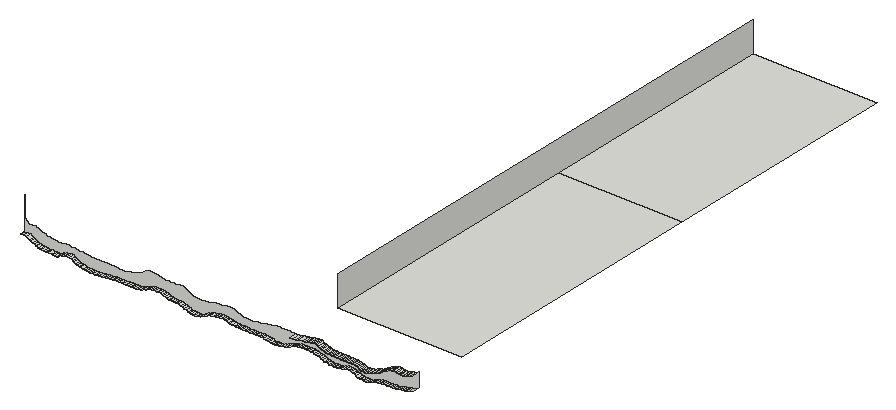
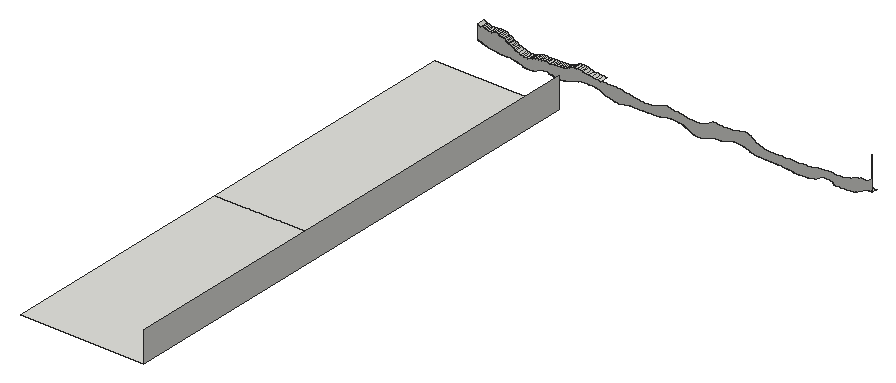
# SketchUp Ruby script. Lengths in inches.
U = 1.inch
M = Sketchup.active_model
def pt(a) = Geom::Point3d.new(a.map { |v| v * U })
def face(e, loops, mat)
  f = e.add_face(loops[0].map { |a| pt(a) })
  loops[1..].each { |l| e.add_face(l.map { |a| pt(a) }).erase! }
  f.material = f.back_material = mat if mat
  f
end
# faces: each face lists its corners as indices into pts; further lists are holes
def faces(e, pts, list, mat = nil) = list.each { |f| face(e, (f[0].is_a?(Array) ? f : [f]).map { |l| l.map { |i| pts[i] } }, mat) }
# xy, xz, yz: faces in a plane at the given z, y or x. An outline is a flat list of corners, or four numbers for a rectangle; further outlines are holes
def ring(l) = l.size == 4 ? [[l[0], l[1]], [l[2], l[1]], [l[2], l[3]], [l[0], l[3]]] : l.each_slice(2).to_a
def flat(e, list, mat, &to3) = list.each { |f| face(e, (f[0].is_a?(Array) ? f : [f]).map { |l| ring(l).map { |u, v| to3.(u, v) } }, mat) }
def xy(e, z, list, mat = nil) = flat(e, list, mat) { |x, y| [x, y, z] }
def xz(e, y, list, mat = nil) = flat(e, list, mat) { |x, z| [x, y, z] }
def yz(e, x, list, mat = nil) = flat(e, list, mat) { |y, z| [x, y, z] }
def lines(e, pts, list) = list.each { |a, b| e.add_line(pt(pts[a]), pt(pts[b])) }
# prism: a flat outline (further loops are holes) pulled along v
def prism(e, loops, v, mat = nil)
  f = face(e, loops, mat); d = Geom::Vector3d.new(v.map { |x| x * U })
  f.pushpull(f.normal.samedirection?(d) ? d.length : -d.length)
end
def box(e, o, s, mat = nil) = prism(e, [[o, [o[0] + s[0], o[1], o[2]], [o[0] + s[0], o[1] + s[1], o[2]], [o[0], o[1] + s[1], o[2]]]], [0, 0, s[2]], mat)
def at(x, y, z, deg = 0) = Geom::Transformation.translation(pt([x, y, z])) * Geom::Transformation.rotation(ORIGIN, Z_AXIS, deg.degrees)
def axes(o, x, y, z) = Geom::Transformation.new([*x, 0, *y, 0, *z, 0, *pt(o).to_a, 1])
def part(name) = M.definitions.add(name)
# library, detail: a bought-in or finely detailed component or shape, given as its bounding box
def library(name, o, s) = part(name).tap { |d| box(d.entities, o, s) }
def detail(e, o, s) = box(e.add_group.entities, o, s)
def put(e, d, t, mat = nil) = e.add_instance(d, t).tap { |i| i.material = mat if mat }
def group(e, t, mat = nil) = e.add_group.tap { |g| g.transformation = t; g.material = mat if mat }.entities
root = M.entities
xy(root,237.65,[[2039.58,566.68,2040.27,568.68],[2040.27,566.68,2040.89,568.68]])
xy(root,238.18,[[2133.53,566.68,2134.21,568.68]])
xy(root,238.33,[[2048.68,566.68,2049.23,568.68],[2049.23,566.68,2049.91,568.68]])
xy(root,238.34,[[2050.59,566.68,2051.52,568.68],[2051.52,566.68,2052.01,568.68],[2052.01,566.68,2052.77,568.68],[2052.77,566.68,2053.4,568.68],[2053.4,566.68,2054.15,568.68],
  [2054.15,566.68,2054.77,568.68],[2054.77,566.68,2055.54,568.68],[2055.54,566.68,2056.16,568.68]])
xy(root,238.62,[[2100.06,566.68,2100.83,568.68],[2100.83,566.68,2101.46,568.68],[2101.46,566.68,2102.22,568.68],[2102.22,566.68,2102.84,568.68],[2102.84,566.68,2103.69,568.68],
  [2103.69,566.68,2104.33,568.68],[2104.33,566.68,2104.95,568.68]])
xy(root,238.625,[[2098.64,566.68,2099.5,568.68]])
xy(root,238.89,[[2154.45,566.68,2155.13,568.68]])
xy(root,238.9,[[2155.89,566.68,2156.51,568.68],[2156.51,566.68,2157.28,568.68]])
xy(root,240.43,[[2122.73,566.68,2123.3,568.68]])
xy(root,241.52,[[2010.28,566.68,2010.34,568.68]])
xy(root,242.28,[[2140.55,565.74,2141.0625,568.68]])
xy(root,242.3,[[2138.79,565.74,2139.46,568.68]])
xy(root,242.33,[[2136.38,565.74,2136.96,568.68]])
xy(root,242.625,[[2115.89,589.83,2164.35,697.21],[2115.89,697.21,2164.35,792.52]])
xz(root,568.68,[[2079.2,236.98,2078.59,237.01,2077.9,237.04,2077.14,237.11,2076.45,237.2,2075.92,237.33,2075.25,237.68,2074.3125,237.96,2073.75,238.28,2072.97,238.43,2072.19,238.78,2071.52,238.79,2070.98,238.8,2070.22,238.83,2069.47,238.875,2068.9,238.94,2068.32,239.04,2067.66,239.29,2067.08,239.53,2066.55,239.7,2065.86,239.92,2065.23,240.11,2064.45,240.27,2063.83,240.25,2063.125,240.23,2062.36,240.19,2061.6875,240.12,2061.03,240.03,2060.39,239.85,2059.84,239.52,2059.28,239.35,2058.69,239.18,2058.18,238.86,2057.49,238.72,2056.67,238.59,2056.16,238.34,2050.59,238.34,2049.91,238.33,2048.68,238.33,2047.96,238.32,2047.11,238.3,2046.48,238.28,2045.73,238.26,2045.1,238.15,2044.34,238.13,2043.79,238.1,2042.9375,237.98,2042.32,237.94,2041.56,237.89,2040.89,237.65,2039.58,237.65,2038.89,237.66,2038.14,237.67,2037.54,237.68,2036.93,237.71,2036.22,237.76,2035.53,237.82,2034.87,237.9,2033.93,238.21,2033.46,238.31,2032.55,238.43,2031.9,238.74,2031.32,239.11,2030.74,239.38,2030.28,239.71,2029.58,240.11,2028.89,240.09,2028.23,240.05,2027.64,239.99,2026.91,239.88,2026.36,239.69,2025.78,239.55,2025.22,238.9375,2024.69,238.77,2023.95,238.79,2023.08,238.8,2022.57,238.82,2021.53,238.92,2020.84,238.93,2020.14,238.94,2019.44,238.97,2018.76,239.03,2018.07,239.09,2017.29,239.19,2016.78,239.52,2016.22,239.64,2015.77,239.86,2014.98,240.2,2014.38,240.59,2013.84,240.85,2012.82,241.55,2011.55,241.69,2010.34,241.52,2010.34,246.2,2011.91,244.96,2013.3,244.9375,2014.55,244.92,2014.77,244.61,2015.33,244.54,2016.09,244.41,2016.76,244.11,2017.28,243.95,2017.94,243.79,2018.46,243.48,2019.1,243.3,2019.6875,243.14,2020.17,243.06,2020.89,242.85,2021.47,242.78,2022.28,242.73,2022.82,242.68,2023.49,242.51,2024.01,242.46,2024.55,242.58,2025.18,242.57,2025.81,242.81,2026.38,242.86,2026.94,242.89,2027.58,242.92,2028.01,242.625,2028.62,242.65,2029.17,242.62,2029.8,242.58,2030.36,242.57,2031,242.48,2031.66,242.38,2032.32,242.34,2032.99,242.24,2034.16,241.96,2034.93,241.89,2035.75,241.83,2036.35,241.78,2037.12,241.75,2037.57,241.74,2038.12,241.72,2039.38,241.7,2040.11,241.69,2040.78,241.68,2041.37,241.68,2041.86,241.67,2042.5625,241.74,2043.13,241.75,2045.13,241.75,2045.62,241.67,2046.15,241.66,2046.76,241.57,2047.3,241.53,2047.92,241.51,2048.47,241.49,2049.17,241.48,2049.83,241.47,2050.4,241.46,2051.11,241.6,2051.84,241.85,2052.51,241.91,2053.41,242.1,2054.18,242.46,2054.88,242.78,2055.65,242.97,2056.18,243.23,2056.58,243.48,2057.1,243.72,2057.4375,244.12,2057.91,244.39,2058.39,244.73,2058.875,244.87,2059.46,244.95,2060.14,245.01,2060.79,244.81,2061.36,244.7,2061.84,244.67,2062.45,244.55,2062.99,244.51,2063.45,244.25,2064.2,244.11,2064.76,244.04,2065.38,243.99,2066.1,243.95,2066.6,243.93,2067.29,243.91,2067.86,243.89,2068.56,243.88,2069.21,243.94,2069.85,243.95,2070.41,244.1,2071.04,244.13,2071.52,244.15,2072.04,244.17,2072.56,244.18,2073.16,243.8,2073.7,243.43,2074.31,243.09,2074.7,242.875,2075.2,242.68,2075.79,242.51,2076.3,242.21,2076.9,242.11,2077.58,241.96,2078.14,241.89,2078.6,241.85,2079.12,241.8125,2079.63,241.79,2080.21,241.78,2080.88,241.91,2081.35,241.93,2082.02,242.09,2082.79,242.2,2083.29,242.24,2083.9,242.42,2084.45,242.47,2085.2,242.71,2085.84,242.78,2086.32,242.82,2087.01,242.85,2087.71,242.87,2088.26,243.02,2088.88,243.05,2089.43,243.29,2090.11,243.35,2090.66,243.39,2091.26,243.42,2092.03,243.14,2092.6,242.9375,2093.15,242.65,2093.77,242.39,2094.53,242.14,2095.17,241.89,2095.66,241.78,2096.71,241.63,2097.48,241.56,2098.08,241.51,2098.53,241.48,2099.05,241.46,2099.92,241.51,2100.64,241.59,2101.58,241.82,2102.36,241.87,2103.125,241.98,2103.74,242.02,2104.39,242.19,2105.09,242.38,2105.58,242.4375,2106.1,242.48,2106.76,242.58,2107.29,242.61,2107.875,242.77,2108.33,242.95,2108.89,243.01,2109.4,243.05,2109.97,243.08,2110.625,243.09,2112.78,243.09,2113.35,243.08,2113.9375,243.07,2114.52,243.07,2115.18,243.0625,2115.79,243.05,2116.47,243.05,2117.74,243.1,2118.91,243.17,2120.05,243.4,2121.3125,243.52,2122.44,243.71,2123.34,243.99,2124.04,244.08,2124.74,244.21,2125.32,244.27,2125.86,244.3,2126.53,244.39,2127.125,244.19,2127.5,243.88,2127.98,243.59,2128.53,243.33,2129.08,243.22,2129.57,242.92,2130.05,242.75,2130.61,242.6,2131.17,242.52,2131.73,242.47,2132.3125,242.43,2132.89,242.4,2133.47,242.39,2134.05,242.37,2134.63,242.36,2135.22,242.35,2136.38,242.33,2136.96,242.33,2137.68,242.32,2138.15,242.3125,2138.79,242.3,2139.46,242.3,2139.91,242.29,2140.55,242.28,2141.0625,242.28,2141.69,242.2,2142.27,241.97,2142.84,241.84,2143.35,241.57,2143.77,241.33,2144.24,241.24,2144.77,241.17,2145.24,241.12,2145.84,241.09,2146.41,241.14,2147.05,241.35,2147.64,241.46,2148.58,241.85,2149.58,242.23,2150.14,242.42,2150.86,242.61,2151.375,242.91,2151.75,243.14,2152.29,243.52,2152.77,243.71,2153.1,244.02,2153.54,244.21,2154.13,244.57,2154.6,244.76,2155.22,245.125,2155.72,245.32,2156.2,245.41,2156.75,245.48,2157.24,245.59,2157.77,245.55,2158.38,245.35,2158.87,245.31,2159.42,245.27,2159.98,245.24,2160.54,245.22,2161.1,245.34,2161.73,245.42,2162.3125,245.52,2162.69,245.76,2163.16,245.9,2164.35,246.43,2164.35,240.89,2162.52,240.1,2161.96,239.96,2161.4375,239.81,2160.75,239.53,2160.2,239.49,2159.48,239.42,2158.68,239.28,2157.91,239.15,2157.28,238.9,2155.89,238.9,2155.13,238.89,2154.45,238.89,2153.77,238.88,2153.23,238.875,2152.47,238.86,2151.73,238.83,2151.16,238.8,2150.58,238.74,2149.92,238.6,2149.35,238.51,2148.82,238.33,2148.13,238.08,2147.45,237.84,2146.76,237.5625,2146.16,237.47,2145.48,237.4,2144.75,237.42,2144.18,237.45,2143.59,237.51,2142.99,237.59,2142.45,237.71,2141.62,238,2140.91,238.33,2140.36,238.57,2139.86,238.86,2139.34,238.96,2138.65,239.02,2137.97,239.125,2137.23,239.04,2136.66,238.66,2136.07,238.61,2135.41,238.55,2134.89,238.27,2134.21,238.18,2133.53,238.18,2132.86,238.11,2132.33,238.15,2131.51,238.19,2130.9375,238.26,2130.37,238.48,2129.71,238.56,2129.14,238.67,2128.62,239.01,2127.9375,239.18,2127.3125,239.5,2126.55,239.65,2125.9375,239.8,2125.18,239.96,2124.53,240.23,2123.95,240.27,2123.3,240.43,2122.73,240.43,2122.15,240.42,2121.625,240.41,2120.93,240.4,2120.24,240.37,2119.55,240.33,2118.87,240.27,2118.19,240.17,2117.57,239.97,2116.92,239.75,2116.18,239.375,2115.39,239.08,2114.51,238.72,2113.76,238.46,2112.54,238.14,2111.42,237.88,2110.77,237.87,2109.9,237.74,2109.19,237.79,2108.42,237.86,2107.79,238.15,2107.02,238.19,2106.4,238.25,2105.64,238.45,2104.95,238.62,2100.06,238.62,2099.5,238.625,2098.64,238.625,2097.95,238.63,2097.33,238.64,2096.55,238.65,2095.88,238.66,2095.19,238.6875,2094.52,238.73,2094.04,238.78,2093.16,238.93,2092.39,239.07,2091.84,239.16,2090.99,239.44,2090.32,239.56,2089.71,239.72,2088.98,239.7,2088.42,239.69,2087.83,239.65,2087.21,239.6,2086.72,239.54,2085.91,239.31,2084.91,239.22,2084.33,239.12,2083.6875,238.76,2083.05,238.51,2082.49,238.375,2082.05,238.02,2081.35,237.74,2080.73,237.43,2079.88,237.22],[2010.28,241.52,2010.34,254.5]])
yz(root,2115.89,[[589.83,242.625,792.52,254.5]])
p = [[2077.14,568.68,237.11],[2077.9,568.68,237.04],[2077.9,566.68,237.04],[2077.14,566.68,237.11],[2078.59,568.68,237.01],[2078.59,566.68,237.01],
  [2079.2,568.68,236.98],[2079.2,566.68,236.98],[2079.88,568.68,237.22],[2079.88,566.68,237.22],[2076.45,568.68,237.2],[2076.45,566.68,237.2],
  [2075.92,568.68,237.33],[2075.92,566.68,237.33],[2080.73,568.68,237.43],[2080.73,566.68,237.43],[2075.25,568.68,237.68],[2075.25,566.68,237.68],
  [2081.35,568.68,237.74],[2081.35,566.68,237.74],[2144.18,568.68,237.45],[2144.75,568.68,237.42],[2144.75,566.68,237.42],[2144.18,566.68,237.45],
  [2145.48,568.68,237.4],[2145.48,566.68,237.4],[2146.16,568.68,237.47],[2146.16,566.68,237.47],[2142.99,568.68,237.59],[2143.59,568.68,237.51],
  [2143.59,566.68,237.51],[2142.99,566.68,237.59],[2146.76,568.68,237.5625],[2146.76,566.68,237.5625],[2040.89,568.68,237.65],[2041.56,568.68,237.89],
  [2041.56,566.68,237.89],[2040.89,566.68,237.65],[2142.45,568.68,237.71],[2142.45,566.68,237.71],[2147.45,568.68,237.84],[2147.45,566.68,237.84],
  [2036.22,568.68,237.76],[2036.93,568.68,237.71],[2036.93,566.68,237.71],[2036.22,566.68,237.76],[2037.54,568.68,237.68],[2037.54,566.68,237.68],
  [2038.14,568.68,237.67],[2038.14,566.68,237.67],[2038.89,568.68,237.66],[2038.89,566.68,237.66],[2039.58,568.68,237.65],[2039.58,566.68,237.65],
  [2074.3125,568.68,237.96],[2074.3125,566.68,237.96],[2082.05,568.68,238.02],[2082.05,566.68,238.02],[2109.19,568.68,237.79],[2109.9,568.68,237.74],
  [2109.9,566.68,237.74],[2109.19,566.68,237.79],[2110.77,568.68,237.87],[2110.77,566.68,237.87],[2141.62,568.68,238],[2141.62,566.68,238],
  [2034.87,568.68,237.9],[2035.53,568.68,237.82],[2035.53,566.68,237.82],[2034.87,566.68,237.9],[2108.42,568.68,237.86],[2108.42,566.68,237.86],
  [2148.13,568.68,238.08],[2148.13,566.68,238.08],[2033.93,568.68,238.21],[2033.93,566.68,238.21],[2042.32,568.68,237.94],[2042.32,566.68,237.94],
  [2042.9375,568.68,237.98],[2042.9375,566.68,237.98],[2107.79,568.68,238.15],[2107.79,566.68,238.15],[2111.42,568.68,237.88],[2111.42,566.68,237.88],
  [2112.54,568.68,238.14],[2112.54,566.68,238.14],[2043.79,568.68,238.1],[2043.79,566.68,238.1],[2073.75,568.68,238.28],[2073.75,566.68,238.28],
  [2082.49,568.68,238.375],[2082.49,566.68,238.375],[2140.91,568.68,238.33],[2140.91,566.68,238.33],[2044.34,568.68,238.13],[2044.34,566.68,238.13],
  [2045.1,568.68,238.15],[2045.1,566.68,238.15],[2107.02,568.68,238.19],[2107.02,566.68,238.19],[2113.76,568.68,238.46],[2113.76,566.68,238.46],
  [2131.51,568.68,238.19],[2132.33,568.68,238.15],[2132.33,566.68,238.15],[2131.51,566.68,238.19],[2132.86,568.68,238.11],[2132.86,566.68,238.11],
  [2133.53,568.68,238.18],[2133.53,566.68,238.18],[2148.82,568.68,238.33],[2148.82,566.68,238.33],[2033.46,568.68,238.31],[2033.46,566.68,238.31],
  [2045.73,568.68,238.26],[2045.73,566.68,238.26],[2106.4,568.68,238.25],[2106.4,566.68,238.25],[2130.9375,568.68,238.26],[2130.9375,566.68,238.26],
  [2134.21,568.68,238.18],[2134.89,568.68,238.27],[2134.89,566.68,238.27],[2134.21,566.68,238.18],[2032.55,568.68,238.43],[2032.55,566.68,238.43],
  [2046.48,568.68,238.28],[2046.48,566.68,238.28],[2047.11,568.68,238.3],[2047.11,566.68,238.3],[2047.96,568.68,238.32],[2047.96,566.68,238.32],
  [2048.68,568.68,238.33],[2048.68,566.68,238.33],[2049.91,568.68,238.33],[2050.59,568.68,238.34],[2050.59,566.68,238.34],[2049.91,566.68,238.33],
  [2056.16,568.68,238.34],[2056.67,568.68,238.59],[2056.67,566.68,238.59],[2056.16,566.68,238.34],[2072.97,568.68,238.43],[2072.97,566.68,238.43],
  [2105.64,568.68,238.45],[2105.64,566.68,238.45],[2130.37,568.68,238.48],[2130.37,566.68,238.48],[2135.41,568.68,238.55],[2135.41,566.68,238.55],
  [2140.36,568.68,238.57],[2140.36,566.68,238.57],[2149.35,568.68,238.51],[2149.35,566.68,238.51],[2031.9,568.68,238.74],[2031.9,566.68,238.74],
  [2072.19,568.68,238.78],[2072.19,566.68,238.78],[2083.05,568.68,238.51],[2083.05,566.68,238.51],[2083.6875,568.68,238.76],[2083.6875,566.68,238.76],
  [2104.95,568.68,238.62],[2104.95,566.68,238.62],[2114.51,568.68,238.72],[2114.51,566.68,238.72],[2129.71,568.68,238.56],[2129.71,566.68,238.56],
  [2136.07,568.68,238.61],[2136.07,566.68,238.61],[2149.92,568.68,238.6],[2149.92,566.68,238.6],[2057.49,568.68,238.72],[2057.49,566.68,238.72],
  [2095.88,568.68,238.66],[2096.55,568.68,238.65],[2096.55,566.68,238.65],[2095.88,566.68,238.66],[2097.33,568.68,238.64],[2097.33,566.68,238.64],
  [2097.95,568.68,238.63],[2097.95,566.68,238.63],[2098.64,568.68,238.625],[2098.64,566.68,238.625],[2099.5,568.68,238.625],[2100.06,568.68,238.62],
  [2100.06,566.68,238.62],[2099.5,566.68,238.625],[2129.14,568.68,238.67],[2129.14,566.68,238.67],[2136.66,568.68,238.66],[2136.66,566.68,238.66],
  [2139.86,568.68,238.86],[2139.86,566.68,238.86],[2150.58,568.68,238.74],[2150.58,566.68,238.74],[2031.32,568.68,239.11],[2031.32,566.68,239.11],
  [2058.18,568.68,238.86],[2058.18,566.68,238.86],[2094.04,568.68,238.78],[2094.52,568.68,238.73],[2094.52,566.68,238.73],[2094.04,566.68,238.78],
  [2095.19,568.68,238.6875],[2095.19,566.68,238.6875],[2115.39,568.68,239.08],[2115.39,566.68,239.08],[2128.62,568.68,239.01],[2128.62,566.68,239.01],
  [2137.23,568.68,239.04],[2137.23,566.68,239.04],[2151.16,568.68,238.8],[2151.16,566.68,238.8],[2021.53,568.68,238.92],[2022.57,568.68,238.82],
  [2022.57,566.68,238.82],[2021.53,566.68,238.92],[2023.08,568.68,238.8],[2023.08,566.68,238.8],[2023.95,568.68,238.79],[2023.95,566.68,238.79],
  [2024.69,568.68,238.77],[2024.69,566.68,238.77],[2025.22,568.68,238.9375],[2025.22,566.68,238.9375],[2069.47,568.68,238.875],[2070.22,568.68,238.83],
  [2070.22,566.68,238.83],[2069.47,566.68,238.875],[2070.98,568.68,238.8],[2070.98,566.68,238.8],[2071.52,568.68,238.79],[2071.52,566.68,238.79],
  [2084.33,568.68,239.12],[2084.33,566.68,239.12],[2093.16,568.68,238.93],[2093.16,566.68,238.93],[2151.73,568.68,238.83],[2151.73,566.68,238.83],
  [2152.47,568.68,238.86],[2152.47,566.68,238.86],[2019.44,568.68,238.97],[2020.14,568.68,238.94],[2020.14,566.68,238.94],[2019.44,566.68,238.97],
  [2020.84,568.68,238.93],[2020.84,566.68,238.93],[2025.78,568.68,239.55],[2025.78,566.68,239.55],[2058.69,568.68,239.18],[2058.69,566.68,239.18],
  [2068.32,568.68,239.04],[2068.9,568.68,238.94],[2068.9,566.68,238.94],[2068.32,566.68,239.04],[2092.39,568.68,239.07],[2092.39,566.68,239.07],
  [2139.34,568.68,238.96],[2139.34,566.68,238.96],[2153.23,568.68,238.875],[2153.23,566.68,238.875],[2153.77,568.68,238.88],[2153.77,566.68,238.88],
  [2154.45,568.68,238.89],[2154.45,566.68,238.89],[2155.13,568.68,238.89],[2155.89,568.68,238.9],[2155.89,566.68,238.9],[2155.13,566.68,238.89],
  [2157.28,568.68,238.9],[2157.91,568.68,239.15],[2157.91,566.68,239.15],[2157.28,566.68,238.9],[2018.07,568.68,239.09],[2018.76,568.68,239.03],
  [2018.76,566.68,239.03],[2018.07,566.68,239.09],[2067.66,568.68,239.29],[2067.66,566.68,239.29],[2127.9375,568.68,239.18],[2127.9375,566.68,239.18],
  [2137.97,568.68,239.125],[2137.97,566.68,239.125],[2138.65,568.68,239.02],[2138.65,566.68,239.02],[2017.29,568.68,239.19],[2017.29,566.68,239.19],
  [2030.74,568.68,239.38],[2030.74,566.68,239.38],[2084.91,568.68,239.22],[2084.91,566.68,239.22],[2091.84,568.68,239.16],[2091.84,566.68,239.16],
  [2116.18,568.68,239.375],[2116.18,566.68,239.375],[2016.78,568.68,239.52],[2016.78,566.68,239.52],[2059.28,568.68,239.35],[2059.28,566.68,239.35],
  [2085.91,568.68,239.31],[2085.91,566.68,239.31],[2090.99,568.68,239.44],[2090.99,566.68,239.44],[2127.3125,568.68,239.5],[2127.3125,566.68,239.5],
  [2158.68,568.68,239.28],[2158.68,566.68,239.28],[2067.08,568.68,239.53],[2067.08,566.68,239.53],[2086.72,568.68,239.54],[2086.72,566.68,239.54],
  [2159.48,568.68,239.42],[2159.48,566.68,239.42],[2030.28,568.68,239.71],[2030.28,566.68,239.71],[2059.84,568.68,239.52],[2059.84,566.68,239.52],
  [2090.32,568.68,239.56],[2090.32,566.68,239.56],[2116.92,568.68,239.75],[2116.92,566.68,239.75],[2160.2,568.68,239.49],[2160.2,566.68,239.49],
  [2016.22,568.68,239.64],[2016.22,566.68,239.64],[2060.39,568.68,239.85],[2060.39,566.68,239.85],[2066.55,568.68,239.7],[2066.55,566.68,239.7],
  [2087.21,568.68,239.6],[2087.21,566.68,239.6],[2126.55,568.68,239.65],[2126.55,566.68,239.65],[2160.75,568.68,239.53],[2160.75,566.68,239.53],
  [2161.4375,568.68,239.81],[2161.4375,566.68,239.81],[2015.77,568.68,239.86],[2015.77,566.68,239.86],[2026.36,568.68,239.69],[2026.36,566.68,239.69],
  [2087.83,568.68,239.65],[2087.83,566.68,239.65],[2088.42,568.68,239.69],[2088.42,566.68,239.69],[2089.71,568.68,239.72],[2089.71,566.68,239.72],
  [2026.91,568.68,239.88],[2026.91,566.68,239.88],[2029.58,568.68,240.11],[2029.58,566.68,240.11],[2065.86,568.68,239.92],[2065.86,566.68,239.92],
  [2088.98,568.68,239.7],[2088.98,566.68,239.7],[2117.57,568.68,239.97],[2117.57,566.68,239.97],[2125.9375,568.68,239.8],[2125.9375,566.68,239.8],
  [2061.03,568.68,240.03],[2061.03,566.68,240.03],[2125.18,568.68,239.96],[2125.18,566.68,239.96],[2161.96,568.68,239.96],[2161.96,566.68,239.96],
  [2014.98,568.68,240.2],[2014.98,566.68,240.2],[2027.64,568.68,239.99],[2027.64,566.68,239.99],[2065.23,568.68,240.11],[2065.23,566.68,240.11],
  [2028.23,568.68,240.05],[2028.23,566.68,240.05],[2028.89,568.68,240.09],[2028.89,566.68,240.09],[2061.6875,568.68,240.12],[2061.6875,566.68,240.12],
  [2118.19,568.68,240.17],[2118.19,566.68,240.17],[2124.53,568.68,240.23],[2124.53,566.68,240.23],[2162.52,568.68,240.1],[2162.52,566.68,240.1],
  [2062.36,568.68,240.19],[2062.36,566.68,240.19],[2064.45,568.68,240.27],[2064.45,566.68,240.27],[2164.35,568.68,240.89],[2164.35,566.68,240.89],
  [2014.38,568.68,240.59],[2014.38,566.68,240.59],[2063.125,568.68,240.23],[2063.125,566.68,240.23],[2063.83,568.68,240.25],[2063.83,566.68,240.25],
  [2118.87,568.68,240.27],[2118.87,566.68,240.27],[2123.95,568.68,240.27],[2123.95,566.68,240.27],[2119.55,568.68,240.33],[2119.55,566.68,240.33],
  [2120.24,568.68,240.37],[2120.24,566.68,240.37],[2123.3,568.68,240.43],[2123.3,566.68,240.43],[2120.93,568.68,240.4],[2120.93,566.68,240.4],
  [2121.625,568.68,240.41],[2121.625,566.68,240.41],[2122.15,568.68,240.42],[2122.15,566.68,240.42],[2122.73,568.68,240.43],[2122.73,566.68,240.43],
  [2013.84,568.68,240.85],[2013.84,566.68,240.85],[2012.82,568.68,241.55],[2012.82,566.68,241.55],[2144.77,568.68,241.17],[2145.24,568.68,241.12],
  [2145.24,565.74,241.12],[2144.77,565.74,241.17],[2145.84,568.68,241.09],[2145.84,565.74,241.09],[2146.41,568.68,241.14],[2146.41,565.74,241.14],
  [2147.05,568.68,241.35],[2147.05,565.74,241.35],[2143.77,568.68,241.33],[2144.24,568.68,241.24],[2144.24,565.74,241.24],[2143.77,565.74,241.33],
  [2143.35,568.68,241.57],[2143.35,565.74,241.57],[2147.64,568.68,241.46],[2147.64,565.74,241.46],[2148.58,568.68,241.85],[2148.58,565.74,241.85],
  [2010.34,568.68,241.52],[2011.55,568.68,241.69],[2011.55,566.68,241.69],[2010.34,566.68,241.52],[2142.84,568.68,241.84],[2142.84,565.74,241.84],
  [2142.27,568.68,241.97],[2142.27,565.74,241.97],[2149.58,568.68,242.23],[2149.58,565.74,242.23],[2141.69,568.68,242.2],[2141.69,565.74,242.2],
  [2141.0625,568.68,242.28],[2141.0625,565.74,242.28],[2150.14,568.68,242.42],[2150.14,565.74,242.42],[2135.22,568.68,242.35],[2135.8,568.68,242.34],
  [2135.8,565.74,242.34],[2135.22,565.74,242.35],[2136.38,568.68,242.33],[2136.38,565.74,242.33],[2136.96,568.68,242.33],[2137.68,568.68,242.32],
  [2137.68,565.74,242.32],[2136.96,565.74,242.33],[2138.15,568.68,242.3125],[2138.15,565.74,242.3125],[2138.79,568.68,242.3],[2138.79,565.74,242.3],
  [2139.46,568.68,242.3],[2139.91,568.68,242.29],[2139.91,565.74,242.29],[2139.46,565.74,242.3],[2140.55,568.68,242.28],[2140.55,565.74,242.28],
  [2131.73,568.68,242.47],[2132.3125,568.68,242.43],[2132.3125,565.74,242.43],[2131.73,565.74,242.47],[2132.89,568.68,242.4],[2132.89,565.74,242.4],
  [2133.47,568.68,242.39],[2133.47,565.74,242.39],[2134.05,568.68,242.37],[2134.05,565.74,242.37],[2134.63,568.68,242.36],[2134.63,565.74,242.36],
  [2150.86,568.68,242.61],[2150.86,565.74,242.61],[2130.61,568.68,242.6],[2131.17,568.68,242.52],[2131.17,565.74,242.52],[2130.61,565.74,242.6],
  [2130.05,568.68,242.75],[2130.05,565.74,242.75],[2151.375,568.68,242.91],[2151.375,565.74,242.91],[2129.57,568.68,242.92],[2129.57,565.74,242.92],
  [2129.08,568.68,243.22],[2129.08,565.74,243.22],[2151.75,568.68,243.14],[2151.75,565.74,243.14],[2116.47,568.68,243.05],[2117.74,568.68,243.1],
  [2117.74,565.74,243.1],[2116.47,565.74,243.05],[2118.91,568.68,243.17],[2118.91,565.74,243.17],[2152.29,568.68,243.52],[2152.29,565.74,243.52],
  [2120.05,568.68,243.4],[2120.05,565.74,243.4],[2128.53,568.68,243.33],[2128.53,565.74,243.33],[2127.98,568.68,243.59],[2127.98,565.74,243.59],
  [2121.3125,568.68,243.52],[2121.3125,565.74,243.52],[2122.44,568.68,243.71],[2122.44,565.74,243.71],[2152.77,568.68,243.71],[2152.77,565.74,243.71],
  [2127.5,568.68,243.88],[2127.5,565.74,243.88],[2123.34,568.68,243.99],[2123.34,565.74,243.99],[2153.1,568.68,244.02],[2153.1,565.74,244.02],
  [2127.125,568.68,244.19],[2127.125,565.74,244.19],[2124.04,568.68,244.08],[2124.04,565.74,244.08],[2153.54,568.68,244.21],[2153.54,565.74,244.21],
  [2124.74,568.68,244.21],[2124.74,565.74,244.21],[2125.32,568.68,244.27],[2125.32,565.74,244.27],[2126.53,568.68,244.39],[2126.53,565.74,244.39],
  [2154.13,568.68,244.57],[2154.13,565.74,244.57],[2125.86,568.68,244.3],[2125.86,565.74,244.3],[2154.6,568.68,244.76],[2154.6,565.74,244.76],
  [2155.22,568.68,245.125],[2155.22,565.74,245.125],[2155.72,568.68,245.32],[2155.72,565.74,245.32],[2159.42,568.68,245.27],[2159.98,568.68,245.24],
  [2159.98,565.74,245.24],[2159.42,565.74,245.27],[2160.54,568.68,245.22],[2160.54,565.74,245.22],[2161.1,568.68,245.34],[2161.1,565.74,245.34],
  [2156.2,568.68,245.41],[2156.2,565.74,245.41],[2157.77,568.68,245.55],[2158.38,568.68,245.35],[2158.38,565.74,245.35],[2157.77,565.74,245.55],
  [2158.87,568.68,245.31],[2158.87,565.74,245.31],[2161.73,568.68,245.42],[2161.73,565.74,245.42],[2156.75,568.68,245.48],[2156.75,565.74,245.48],
  [2162.3125,568.68,245.52],[2162.3125,565.74,245.52],[2157.24,568.68,245.59],[2157.24,565.74,245.59],[2162.69,568.68,245.76],[2162.69,565.74,245.76],
  [2163.16,568.68,245.9],[2163.16,565.74,245.9],[2164.35,568.68,246.43],[2164.35,565.74,246.43]]
faces(root,p,[[0,1,2,3],[1,4,5,2],[4,6,7,5],[6,8,9,7],[10,0,3,11],[12,10,11,13],[8,14,15,9],[16,12,13,17],
  [14,18,19,15],[20,21,22,23],[21,24,25,22],[24,26,27,25],[28,29,30,31],[29,20,23,30],[26,32,33,27],[34,35,36,37],
  [38,28,31,39],[32,40,41,33],[42,43,44,45],[43,46,47,44],[46,48,49,47],[48,50,51,49],[50,52,53,51],[54,16,17,55],
  [18,56,57,19],[58,59,60,61],[59,62,63,60],[64,38,39,65],[66,67,68,69],[67,42,45,68],[70,58,61,71],[40,72,73,41],
  [74,66,69,75],[35,76,77,36],[76,78,79,77],[80,70,71,81],[62,82,83,63],[82,84,85,83],[78,86,87,79],[88,54,55,89],
  [56,90,91,57],[92,64,65,93],[86,94,95,87],[94,96,97,95],[98,80,81,99],[84,100,101,85],[102,103,104,105],[103,106,107,104],
  [106,108,109,107],[72,110,111,73],[112,74,75,113],[96,114,115,97],[116,98,99,117],[118,102,105,119],[120,121,122,123],[124,112,113,125],
  [114,126,127,115],[126,128,129,127],[128,130,131,129],[130,132,133,131],[134,135,136,137],[138,139,140,141],[142,88,89,143],[144,116,117,145],
  [146,118,119,147],[121,148,149,122],[150,92,93,151],[110,152,153,111],[154,124,125,155],[156,142,143,157],[90,158,159,91],[158,160,161,159],
  [162,144,145,163],[100,164,165,101],[166,146,147,167],[148,168,169,149],[152,170,171,153],[139,172,173,140],[174,175,176,177],[175,178,179,176],
  [178,180,181,179],[180,182,183,181],[184,185,186,187],[188,166,167,189],[168,190,191,169],[192,150,151,193],[170,194,195,171],[196,154,155,197],
  [172,198,199,173],[200,201,202,203],[201,204,205,202],[204,174,177,205],[164,206,207,165],[208,188,189,209],[190,210,211,191],[194,212,213,195],
  [214,215,216,217],[215,218,219,216],[218,220,221,219],[220,222,223,221],[222,224,225,223],[226,227,228,229],[227,230,231,228],[230,232,233,231],
  [232,156,157,233],[160,234,235,161],[236,200,203,237],[212,238,239,213],[238,240,241,239],[242,243,244,245],[243,246,247,244],[246,214,217,247],
  [224,248,249,225],[198,250,251,199],[252,253,254,255],[253,226,229,254],[256,236,237,257],[258,192,193,259],[240,260,261,241],[260,262,263,261],
  [262,264,265,263],[266,267,268,269],[270,271,272,273],[274,275,276,277],[275,242,245,276],[278,252,255,279],[280,208,209,281],[210,282,283,211],
  [282,284,285,283],[284,258,259,285],[286,274,277,287],[288,196,197,289],[234,290,291,235],[292,256,257,293],[206,294,295,207],[296,286,287,297],
  [250,298,299,251],[290,300,301,291],[302,292,293,303],[304,280,281,305],[271,306,307,272],[308,278,279,309],[300,310,311,301],[306,312,313,307],
  [314,288,289,315],[298,316,317,299],[318,302,303,319],[294,320,321,295],[312,322,323,313],[324,296,297,325],[316,326,327,317],[328,308,309,329],
  [310,330,331,311],[332,304,305,333],[322,334,335,323],[334,336,337,335],[338,324,325,339],[248,340,341,249],[330,342,343,331],[342,344,345,343],
  [346,318,319,347],[340,348,349,341],[350,314,315,351],[352,328,329,353],[344,354,355,345],[354,346,347,355],[320,356,357,321],[358,332,333,359],
  [326,360,361,327],[362,358,359,363],[336,364,365,337],[366,338,339,367],[348,368,369,349],[370,352,353,371],[368,372,373,369],[372,374,375,373],
  [360,376,377,361],[356,378,379,357],[380,362,363,381],[364,382,383,365],[374,350,351,375],[376,384,385,377],[386,370,371,387],[382,388,389,383],
  [390,366,367,391],[384,392,393,385],[392,394,395,393],[378,396,397,379],[398,380,381,399],[394,386,387,395],[396,400,401,397],[400,402,403,401],
  [404,398,399,405],[402,406,407,403],[406,408,409,407],[408,410,411,409],[410,412,413,411],[414,390,391,415],[416,414,415,417],[418,419,420,421],
  [419,422,423,420],[422,424,425,423],[424,426,427,425],[428,429,430,431],[429,418,421,430],[432,428,431,433],[426,434,435,427],[434,436,437,435],
  [438,439,440,441],[442,432,433,443],[439,416,417,440],[444,442,443,445],[436,446,447,437],[448,444,445,449],[450,448,449,451],[446,452,453,447],
  [454,455,456,457],[455,458,459,456],[460,461,462,463],[461,464,465,462],[464,466,467,465],[468,469,470,471],[469,472,473,470],[474,475,476,477],
  [475,478,479,476],[478,480,481,479],[480,482,483,481],[482,484,485,483],[484,454,457,485],[452,486,487,453],[488,489,490,491],[489,474,477,490],
  [492,488,491,493],[486,494,495,487],[496,492,493,497],[498,496,497,499],[494,500,501,495],[502,503,504,505],[503,506,507,504],[500,508,509,501],
  [506,510,511,507],[512,498,499,513],[514,512,513,515],[510,516,517,511],[516,518,519,517],[508,520,521,509],[522,514,515,523],[518,524,525,519],
  [520,526,527,521],[528,522,523,529],[524,530,531,525],[526,532,533,527],[530,534,535,531],[534,536,537,535],[538,528,529,539],[532,540,541,533],
  [536,542,543,537],[542,538,539,543],[540,544,545,541],[544,546,547,545],[546,548,549,547],[550,551,552,553],[551,554,555,552],[554,556,557,555],
  [548,558,559,549],[560,561,562,563],[561,564,565,562],[564,550,553,565],[556,566,567,557],[558,568,569,559],[566,570,571,567],[568,572,573,569],
  [570,574,575,571],[572,560,563,573],[574,576,577,575],[576,578,579,577]])
